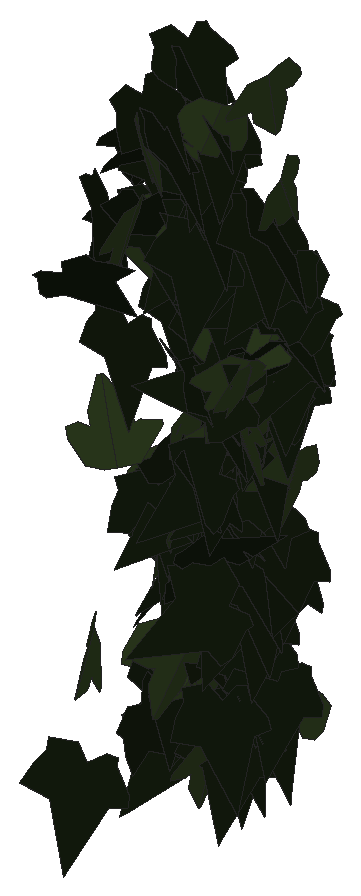
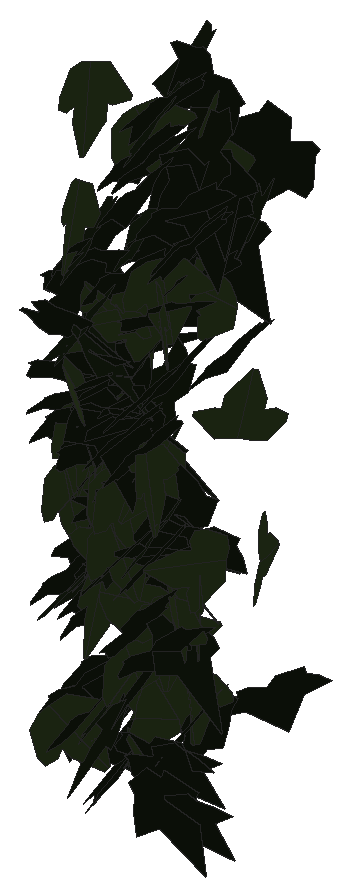
# SketchUp Ruby script. Lengths in inches.
U = 1.inch
M = Sketchup.active_model
def pt(a) = Geom::Point3d.new(a.map { |v| v * U })
def face(e, loops, mat)
  f = e.add_face(loops[0].map { |a| pt(a) })
  loops[1..].each { |l| e.add_face(l.map { |a| pt(a) }).erase! }
  f.material = f.back_material = mat if mat
  f
end
# faces: each face lists its corners as indices into pts; further lists are holes
def faces(e, pts, list, mat = nil) = list.each { |f| face(e, (f[0].is_a?(Array) ? f : [f]).map { |l| l.map { |i| pts[i] } }, mat) }
# xy, xz, yz: faces in a plane at the given z, y or x. An outline is a flat list of corners, or four numbers for a rectangle; further outlines are holes
def ring(l) = l.size == 4 ? [[l[0], l[1]], [l[2], l[1]], [l[2], l[3]], [l[0], l[3]]] : l.each_slice(2).to_a
def flat(e, list, mat, &to3) = list.each { |f| face(e, (f[0].is_a?(Array) ? f : [f]).map { |l| ring(l).map { |u, v| to3.(u, v) } }, mat) }
def xy(e, z, list, mat = nil) = flat(e, list, mat) { |x, y| [x, y, z] }
def xz(e, y, list, mat = nil) = flat(e, list, mat) { |x, z| [x, y, z] }
def yz(e, x, list, mat = nil) = flat(e, list, mat) { |y, z| [x, y, z] }
def lines(e, pts, list) = list.each { |a, b| e.add_line(pt(pts[a]), pt(pts[b])) }
# prism: a flat outline (further loops are holes) pulled along v
def prism(e, loops, v, mat = nil)
  f = face(e, loops, mat); d = Geom::Vector3d.new(v.map { |x| x * U })
  f.pushpull(f.normal.samedirection?(d) ? d.length : -d.length)
end
def box(e, o, s, mat = nil) = prism(e, [[o, [o[0] + s[0], o[1], o[2]], [o[0] + s[0], o[1] + s[1], o[2]], [o[0], o[1] + s[1], o[2]]]], [0, 0, s[2]], mat)
def at(x, y, z, deg = 0) = Geom::Transformation.translation(pt([x, y, z])) * Geom::Transformation.rotation(ORIGIN, Z_AXIS, deg.degrees)
def axes(o, x, y, z) = Geom::Transformation.new([*x, 0, *y, 0, *z, 0, *pt(o).to_a, 1])
def part(name) = M.definitions.add(name)
# library, detail: a bought-in or finely detailed component or shape, given as its bounding box
def library(name, o, s) = part(name).tap { |d| box(d.entities, o, s) }
def detail(e, o, s) = box(e.add_group.entities, o, s)
def put(e, d, t, mat = nil) = e.add_instance(d, t).tap { |i| i.material = mat if mat }
def group(e, t, mat = nil) = e.add_group.tap { |g| g.transformation = t; g.material = mat if mat }.entities
root = M.entities
M.materials.add("efeu1").color = [18, 25, 13]
M.materials.add("efeu2").color = [43, 57, 29]
c1 = part("ivyleaf_9")
p = [[1.54,2.16,1.25],[1.36,2.04,1.19],[-0.21,0.99,0.68],[-0.71,1.11,0.82],[-0.85,0.86,0.67],[-0.8,0.17,0.21],
  [-0.9,-0.01,0.1],[-0.67,-0.16,-0.02],[-0.08,-0.08,-0.05],[-0.03,-0.6,-0.4],[0.65,-0.88,-0.66],[0.83,-0.6,-0.49],
  [1.29,-0.42,-0.43],[1.8125,-0.07,-0.26],[1.21,0.44,0.15]]
faces(c1.entities,p,[[0,1,2,3,4,5,6,7,8,9,10,11,12,13,14]],"efeu1")
c2 = part("ivyleaf_10")
p = [[0,0.5,-0.03],[-0.0625,2.02,-0.43],[-0.19,2.01,-0.46],[-0.54,1.05,-0.29],[-0.52,0.625,-0.18],[-0.83,0.76,-0.28],
  [-1.16,0.64,-0.33],[-1.15,0.33,-0.24],[-0.77,-0.39,0.02],[-0.3,-0.51,0.16],[0.04,-0.48,0.23],[-0.02,2.01,-0.4375],
  [-0.06,2.01,-0.43],[0.04,-0.49,0.23],[0.67,-0.49,0.14],[1.38,0.36,-0.2],[1.375,0.51,-0.24],[0.81,0.65,-0.19],
  [0.62,0.59,-0.15],[0.6,1.09,-0.28],[0.5,1.23,-0.31]]
faces(c2.entities,p,[[0,1,2,3,4,5,6,7,8,9,10],[11,12,0,13,14,15,16,17,18,19,20]],"efeu2")
put(root,c1,axes([13.8,220.49,231.59],[0.40217,0.29091,0.06026],[0.04847,0.03581,-0.49636],[-0.2931,0.40508,0.0006]))
put(root,c2,axes([13.58,221.33,225.61],[-0.05871,0.16785,-0.46731],[0.09367,-0.45837,-0.17641],[-0.48763,-0.10826,0.02238]))
put(root,c1,axes([13.43,221.35,223.65],[-0.19492,-0.45767,-0.05048],[0.01902,0.04677,-0.49744],[0.46005,-0.19584,-0.00082]))
put(root,c1,axes([14.31,221.9375,233.21],[0.2577,-0.40771,0.13176],[0.06772,-0.11306,-0.48232],[0.42309,0.26643,-0.00305]))
put(root,c2,axes([13.76,221.86,231.8],[0.12939,-0.48149,0.03781],[0.01026,-0.0364,-0.49857],[0.48286,0.1298,0.00046]))
put(root,c1,axes([14.9375,222.37,226.15],[-0.39937,-0.19145,0.23205],[-0.21041,-0.09789,-0.44289],[0.21501,-0.4514,-0.00238]))
put(root,c1,axes([12.92,222.48,231.29],[0.01902,-0.28272,0.41195],[0.05223,-0.40887,-0.28302],[0.4969,0.0538,0.01398]))
put(root,c2,axes([13.3,222.09,228.09],[0.35478,0.34849,0.05186],[-0.03906,-0.03425,0.49729],[0.35015,-0.35691,0.00292]))
put(root,c1,axes([13.72,222.21,233.43],[-0.10131,-0.11608,-0.47567],[0.43069,0.20993,-0.14296],[0.23291,-0.4387,0.05745]))
put(root,c2,axes([13.75,222.17,232.93],[-0.27113,0.40326,0.11775],[-0.0681,0.0961,-0.48593],[-0.41455,-0.27954,0.00281]))
put(root,c1,axes([13.07,222.68,229.56],[0.02778,-0.49386,0.07302],[0.02494,-0.07167,-0.49421],[0.4986,0.0311,0.02065]))
put(root,c1,axes([14.53,222.69,227.84],[-0.49906,0.01137,0.02846],[-0.02831,0.00672,-0.49915],[-0.01173,-0.49983,-0.00606]))
put(root,c1,axes([14.83,222.87,229.07],[-0.32268,0.03658,0.38018],[-0.34474,-0.24216,-0.26929],[0.16443,-0.43592,0.1815]))
put(root,c1,axes([14.16,222.89,231.09],[-0.08668,-0.49241,0.00475],[-0.00072,-0.0047,-0.49998],[0.49243,-0.08668,0.0001]))
put(root,c2,axes([14.82,222.86,229.375],[-0.12898,-0.42351,0.23239],[-0.01836,-0.23606,-0.44039],[0.48273,-0.12213,0.04534]))
put(root,c2,axes([13.875,222.85,224.9],[-0.13773,-0.43388,0.20682],[-0.0089,-0.2128,-0.45237],[0.48057,-0.12829,0.05089]))
put(root,c1,axes([13.18,222.78,231.4],[-0.01059,0.33099,-0.37461],[-0.03271,-0.37435,-0.32984],[-0.49882,0.01752,0.02958]))
put(root,c1,axes([14.3125,222.82,229.18],[0.24712,-0.43369,-0.02911],[-0.0123,0.0265,-0.49915],[0.43449,0.24742,0.00243]))
put(root,c1,axes([14.36,222.34,226.53],[0.02979,0.31156,-0.38992],[-0.03442,0.39097,0.30977],[0.49792,0.00839,0.04475]))
put(root,c1,axes([14.48,222.91,224.27],[-0.01662,-0.48072,-0.13651],[0.01341,0.1361,-0.48093],[0.49954,-0.01964,0.00837]))
put(root,c1,axes([14.125,223.16,227.42],[0.03693,-0.39453,0.30493],[0.08476,-0.29635,-0.39369],[0.49138,0.08077,0.04499]))
put(root,c2,axes([14.82,222.96,229.27],[0.10134,-0.48408,0.07345],[0.04823,-0.06477,-0.49344],[0.48724,0.10709,0.03356]))
put(root,c1,axes([13.14,222.84,232.71],[0.45503,-0.16343,0.12743],[0.12074,-0.04079,-0.48348],[0.16842,0.47077,0.00234]))
put(root,c2,axes([14.2,223.11,232.9],[-0.27405,-0.36356,0.2067],[-0.03242,-0.22791,-0.44385],[0.41695,-0.25668,0.10134]))
put(root,c1,axes([13.32,222.7,223.94],[0.12955,-0.17125,-0.45154],[-0.27108,0.36112,-0.21473],[0.39967,0.30044,0.00072]))
put(root,c2,axes([14.22,223,223.52],[-0.00411,-0.49998,0.00247],[0.00009,-0.00247,-0.49999],[0.49998,-0.00411,0.00011]))
put(root,c1,axes([14.42,223.29,225.77],[-0.15318,-0.46276,0.11131],[-0.00387,-0.11572,-0.48641],[0.47594,-0.14987,0.03187]))
put(root,c1,axes([13.64,223.17,228.84],[0.2707,-0.28854,0.30573],[0.20662,-0.22535,-0.39563],[0.3661,0.34053,-0.00277]))
put(root,c1,axes([13.97,223.33,232.49],[-0.07643,-0.4726,0.14423],[0.01277,-0.14779,-0.47749],[0.49396,-0.0693,0.03466]))
put(root,c1,axes([14.39,223.21,230.55],[-0.07448,-0.48829,-0.07762],[0.01205,0.07668,-0.49394],[0.49427,-0.07545,0.00035]))
put(root,c1,axes([13.98,223.13,226.47],[-0.46616,0.15472,-0.09356],[0.07969,-0.05644,-0.49037],[-0.16231,-0.4721,0.02796]))
put(root,c1,axes([14.8,223.07,229.54],[-0.05792,0.39795,-0.29712],[-0.01346,-0.30028,-0.39956],[-0.49645,-0.03828,0.0455]))
put(root,c1,axes([13.9375,223.37,231.42],[0.12592,-0.42098,0.23857],[0.09317,-0.22081,-0.43882],[0.47483,0.15497,0.02283]))
put(root,c1,axes([13.22,222.99,232.48],[0.14415,0.41585,-0.23726],[-0.11216,-0.21156,-0.43894],[-0.46545,0.17977,0.03229]))
put(root,c1,axes([13.2,223.1875,226.9375],[-0.22781,-0.27437,-0.35046],[0.25165,0.24533,-0.35565],[0.36712,-0.33843,0.02632]))
put(root,c2,axes([12.81,223.1875,230.6875],[0.03293,-0.00362,-0.4989],[0.48507,-0.11672,0.03286],[-0.11671,-0.48617,-0.00418]))
put(root,c1,axes([14.33,223.4,223.53],[-0.1431,-0.47844,-0.0248],[0.00712,0.02375,-0.49938],[0.47903,-0.14328,0.00002]))
put(root,c2,axes([14.54,223.125,228.58],[-0.42208,0.24059,-0.11818],[0.11016,-0.04527,-0.48561],[-0.24437,-0.43597,-0.01479]))
put(root,c1,axes([13.16,223.02,232.26],[0.02208,0.48811,-0.10612],[-0.0255,-0.10498,-0.48819],[-0.49886,0.02697,0.02025]))
put(root,c1,axes([13.13,223.47,224.07],[0.0721,-0.47323,0.14443],[0.01853,-0.14327,-0.47868],[0.49443,0.07438,-0.00313]))
put(root,c1,axes([13.625,223.48,226.87],[-0.43349,-0.22149,0.11413],[-0.08849,-0.07725,-0.48601],[0.23293,-0.44156,0.02777]))
put(root,c1,axes([13.6,223.47,226.4],[-0.23787,-0.43953,-0.01522],[0.00627,0.01391,-0.49977],[0.43975,-0.23795,-0.0011]))
put(root,c2,axes([13.33,223.48,226.14],[0.1681,-0.30768,0.35648],[0.23999,-0.26969,-0.34594],[0.40515,0.28741,0.05702]))
put(root,c2,axes([14.22,223.02,229.86],[-0.00451,-0.13108,-0.48249],[0.43338,0.23958,-0.06914],[0.24931,-0.41883,0.11145]))
put(root,c1,axes([13.01,223.39,231.07],[0.03277,-0.48026,-0.1352],[0.00898,0.13604,-0.48105],[0.49884,0.0291,0.01754]))
put(root,c1,axes([13.97,223.51,232.7],[0.00664,-0.49941,0.02346],[0.00257,-0.02343,-0.49944],[0.49995,0.00676,0.00225]))
put(root,c1,axes([13.66,223.47,233.3],[0.23133,-0.44022,0.0519],[0.01667,-0.04986,-0.49723],[0.44295,0.23178,-0.00839]))
put(root,c2,axes([14.54,223.15,229.6],[0.44429,0.0906,-0.21072],[0.18189,0.14069,0.44399],[0.13974,-0.47117,0.09205]))
put(root,c2,axes([13.21,223.35,224.625],[0.4042,0.29343,-0.0228],[-0.01842,-0.01343,-0.49948],[-0.29374,0.40462,-0.00005]))
put(root,c1,axes([14.61,223.625,225.58],[-0.00863,-0.48833,0.10704],[-0.009,-0.10689,-0.48836],[0.49984,-0.01036,-0.00695]))
put(root,c1,axes([14.47,223.47,226.4],[0.20512,-0.45452,-0.03653],[-0.01286,0.03428,-0.49866],[0.45581,0.20551,0.00237]))
put(root,c1,axes([13.52,223.42,233.67],[0.12425,-0.46195,-0.14548],[0.0302,0.15729,-0.47365],[0.48337,0.10892,0.06699]))
put(root,c2,axes([13.12,223.27,226.23],[0.26637,-0.35799,-0.22559],[-0.05657,0.23404,-0.43821],[0.41934,0.25897,0.08418]))
put(root,c1,axes([13.16,223.69,229.68],[0.07704,-0.48639,0.08656],[0.01603,-0.0851,-0.49244],[0.49377,0.07865,0.00248]))
put(root,c2,axes([13.97,223.62,224.86],[-0.18934,-0.43701,0.15222],[-0.01224,-0.15968,-0.47366],[0.4626,-0.18309,0.04978]))
put(root,c1,axes([14.99,223.86,230.32],[-0.25434,-0.23956,0.35766],[-0.26721,-0.23784,-0.34932],[0.33751,-0.36884,-0.00704]))
put(root,c1,axes([12.88,223.68,231.85],[0.05867,-0.49537,-0.0341],[0.00406,0.03481,-0.49877],[0.49653,0.05825,0.00811]))
put(root,c1,axes([13.09,223.7,232.24],[-0.08759,-0.48806,-0.06424],[0.00979,0.06351,-0.49585],[0.49217,-0.08812,-0.00157]))
put(root,c1,axes([14.82,223.83,230.78],[-0.30877,-0.37835,0.1073],[-0.04319,-0.10297,-0.48737],[0.39089,-0.31024,0.03091]))
put(root,c1,axes([14.4,223.78,227.33],[-0.43744,-0.19281,0.14653],[-0.1209,-0.08828,-0.47706],[0.20983,-0.45281,0.03061]))
put(root,c1,axes([13.8,223.7,232.29],[0.06384,-0.49524,-0.02571],[-0.00083,0.02582,-0.49933],[0.49591,0.0638,0.00248]))
put(root,c1,axes([14.57,223.73,231.27],[0.01078,-0.49938,-0.02236],[-0.01016,0.02214,-0.49941],[0.49978,0.01122,-0.00967]))
put(root,c2,axes([14.82,223.46,233.5],[-0.12814,-0.46412,-0.13481],[0.02634,0.13256,-0.48139],[0.48258,-0.13047,-0.00953]))
put(root,c1,axes([14.44,223.71,225.98],[0.03777,-0.49587,-0.05183],[0.00194,0.05212,-0.49727],[0.49857,0.03736,0.00586]))
put(root,c1,axes([14.3125,223.73,224.88],[-0.04806,-0.48879,-0.09366],[0.00931,0.0932,-0.49115],[0.4976,-0.04896,0.00015]))
put(root,c2,axes([13.52,223.875,224.29],[0.01584,0.20118,-0.45747],[-0.18745,-0.42189,-0.19203],[-0.46326,0.17759,0.06206]))
put(root,c1,axes([13.47,223.79,227.07],[0.18622,-0.4485,0.11902],[0.04437,-0.11045,-0.48563],[0.4619,0.19143,-0.00134]))
put(root,c1,axes([13.33,223.36,227.04],[0.07028,-0.00591,0.495],[0.47915,0.12645,-0.06652],[-0.1244,0.48371,0.02343]))
put(root,c1,axes([13.66,223.5,224.92],[0.26332,-0.33557,-0.26087],[-0.13906,0.22198,-0.4259],[0.40165,0.29685,0.02357]))
put(root,c2,axes([14.14,223.68,225.9],[0.05906,0.01763,-0.49619],[-0.4942,-0.04594,-0.06045],[-0.04772,0.49757,0.012]))
put(root,c1,axes([13.22,223.53,225.54],[-0.21933,0.43648,-0.10667],[0.01729,-0.11042,-0.48735],[-0.44899,-0.21747,0.03335]))
put(root,c1,axes([13.39,223.95,230.59],[-0.33004,-0.35694,0.1169],[0.00234,-0.15757,-0.47452],[0.37559,-0.31268,0.10568]))
put(root,c1,axes([14.0625,223.75,227.49],[-0.03503,-0.48074,-0.13289],[0.0501,0.12916,-0.48043],[0.49625,-0.04697,0.03912]))
put(root,c1,axes([14.7,223.89,224.36],[-0.10382,-0.4889,0.0141],[-0.00248,-0.01389,-0.4998],[0.4891,-0.10385,0.00046]))
put(root,c1,axes([13.99,223.93,223.28],[0.08024,-0.46634,0.16152],[0.01253,-0.16166,-0.47298],[0.49336,0.07995,-0.01425]))
put(root,c1,axes([13.12,223.875,223.02],[-0.44422,-0.2295,0.00212],[-0.00164,-0.00143,-0.5],[0.2295,-0.44422,0.00052]))
put(root,c2,axes([13.36,223.58,225.77],[-0.49094,-0.01072,0.09416],[-0.09429,0.00527,-0.491],[0.00953,-0.49986,-0.0072]))
put(root,c1,axes([13.58,223.96,229.22],[-0.01071,-0.4769,0.14984],[0.0416,-0.1502,-0.47509],[0.49815,0.00229,0.04289]))
put(root,c1,axes([14.53,223.79,231.34],[0.27326,-0.41605,0.04726],[0.01506,-0.04663,-0.49759],[0.41845,0.27337,-0.01295]))
put(root,c1,axes([14.4,223.9,227.8],[0.11736,-0.47512,0.10238],[0.03183,-0.09759,-0.48935],[0.48499,0.12138,0.00734]))
put(root,c1,axes([14.61,223.72,229.77],[-0.39206,0.29048,-0.10915],[0.05707,-0.10538,-0.48543],[-0.30501,-0.39309,0.04948]))
put(root,c2,axes([14.02,223.83,227.73],[-0.28066,-0.37112,0.18302],[-0.04172,-0.19465,-0.45866],[0.41169,-0.27273,0.07829]))
put(root,c1,axes([14.625,223.98,228.61],[-0.42637,-0.24126,0.10001],[-0.0508,-0.11119,-0.48483],[0.25618,-0.42359,0.07031]))
put(root,c1,axes([13.93,224.01,226.64],[-0.33682,-0.3631,0.06865],[-0.00063,-0.09232,-0.4914],[0.36953,-0.33111,0.06173]))
put(root,c2,axes([12.82,223.35,226.7],[0.01852,0.04871,-0.49728],[0.294,0.40129,0.05026],[0.404,-0.29426,-0.01378]))
put(root,c1,axes([14.3125,223.96,228.6],[-0.11677,-0.48596,0.0144],[-0.01172,-0.01199,-0.49972],[0.48603,-0.11704,-0.00859]))
put(root,c1,axes([14.32,223.77,226.75],[-0.11951,-0.4109,-0.25862],[0.07997,0.24604,-0.42787],[0.47888,-0.14363,0.00691]))
put(root,c1,axes([12.78,223.86,231.86],[0.11637,-0.48047,-0.07486],[-0.00519,0.07574,-0.4942],[0.48624,0.1158,0.01264]))
put(root,c2,axes([13.56,223.49,228.1],[-0.10261,-0.32946,-0.36184],[0.14529,0.33253,-0.34397],[0.46729,-0.17573,0.0275]))
put(root,c1,axes([14.07,223.625,226.6875],[0.43188,-0.22495,-0.11347],[-0.05725,0.13167,-0.47894],[0.24535,0.42669,0.08798]))
put(root,c2,axes([14.25,223.6875,228.6],[-0.45999,-0.18522,-0.0641],[0.0585,0.02633,-0.49587],[0.18706,-0.46368,-0.00255]))
put(root,c1,axes([14.5,223.88,224.01],[0.08757,-0.48469,-0.08607],[-0.01957,0.08392,-0.49252],[0.49188,0.08963,-0.00427]))
put(root,c1,axes([13.22,224.02,223.81],[-0.43498,-0.24522,0.02564],[-0.02247,-0.01236,-0.49934],[0.24553,-0.43556,-0.00027]))
put(root,c1,axes([14.8125,224.08,229.42],[-0.33994,-0.36666,0.00079],[0.056,-0.05298,-0.49402],[0.36236,-0.33579,0.07709]))
put(root,c1,axes([14.21,223.65,224.12],[0.40294,-0.14969,-0.25541],[-0.22789,0.1185,-0.42898],[0.18896,0.46211,0.02728]))
put(root,c1,axes([14.65,224.16,225.95],[-0.04895,-0.41588,0.27322],[0.06452,-0.27753,-0.41087],[0.4934,-0.00497,0.08083]))
put(root,c1,axes([13.6,224.21,225.73],[-0.18554,-0.34655,0.30899],[-0.0977,-0.29616,-0.39082],[0.45391,-0.2054,0.04219]))
put(root,c1,axes([14.54,223.85,230.07],[0.30917,-0.38808,-0.06173],[-0.00582,0.07401,-0.49446],[0.39291,0.30646,0.04125]))
put(root,c2,axes([13.22,223.91,231.22],[-0.36911,-0.32634,0.0852],[0.00701,-0.1337,-0.48174],[0.3372,-0.35444,0.10328]))
put(root,c1,axes([13.82,223.9375,228.61],[0.12426,-0.47795,-0.07827],[0.01517,0.0846,-0.49256],[0.48408,0.12003,0.03553]))
put(root,c2,axes([13.85,223.95,227.6875],[-0.20201,-0.44429,0.10863],[0.02114,-0.1277,-0.48296],[0.45689,-0.19053,0.07037]))
put(root,c1,axes([13.86,223.97,223.52],[0.16845,-0.46881,-0.04288],[-0.01071,0.04171,-0.49814],[0.47065,0.16874,0.00401]))
put(root,c2,axes([14.39,223.71,225.98],[-0.02638,-0.43565,-0.24394],[0.05084,0.24067,-0.43531],[0.49671,-0.04777,0.0316]))
put(root,c1,axes([14.67,224.13,226.28],[-0.03332,-0.49542,0.05869],[0.00518,-0.05916,-0.49646],[0.49886,-0.03248,0.00907]))
put(root,c1,axes([13.28,224.06,224.01],[-0.39754,-0.25166,-0.16922],[0.16474,0.05503,-0.46886],[0.25461,-0.42853,0.03917]))
put(root,c1,axes([14.13,223.72,228.84],[0.08879,0.46068,-0.17289],[-0.08889,-0.15778,-0.46605],[-0.48396,0.1135,0.05388]))
put(root,c2,axes([13.49,223.85,228.24],[0.07923,-0.48306,-0.10188],[-0.02362,0.09936,-0.48946],[0.49312,0.08237,-0.00707]))
put(root,c2,axes([13.34,223.84,230.88],[0.30776,-0.3712,-0.13226],[-0.04593,0.13289,-0.47982],[0.39137,0.30749,0.0477]))
put(root,c2,axes([14.82,223.96,227.55],[-0.08902,-0.48914,0.05311],[0.00344,-0.05459,-0.497],[0.492,-0.08813,0.01308]))
put(root,c1,axes([13.43,224.04,228.56],[0.09739,-0.48852,-0.04319],[-0.00912,0.04222,-0.49813],[0.49034,0.09781,-0.00069]))
put(root,c1,axes([13.18,223.92,223.43],[-0.148,0.3929,-0.27152],[0.09731,-0.25349,-0.41985],[-0.46757,-0.17712,-0.00144]))
put(root,c2,axes([14.06,223.93,226.82],[-0.09124,-0.49029,0.03591],[0.02918,0.03106,0.49818],[-0.49074,0.093,0.02294]))
put(root,c2,axes([14.75,223.88,228.43],[-0.02645,-0.49427,-0.07072],[0.01343,0.07009,-0.49488],[0.49912,-0.02808,0.00957]))
put(root,c1,axes([14.57,224.15,229.09],[-0.10066,-0.48892,-0.02868],[0.11257,0.0054,-0.48713],[0.47665,-0.10453,0.10899]))
put(root,c1,axes([13.125,224.22,225.61],[-0.18548,-0.45683,0.08308],[-0.00561,-0.08725,-0.4923],[0.46429,-0.18355,0.02724]))
put(root,c1,axes([14.24,224.24,228.46],[-0.2255,-0.43273,0.10904],[-0.05327,-0.09519,-0.48796],[0.44307,-0.23169,-0.00317]))
put(root,c2,axes([14.79,224.14,223.91],[-0.27535,-0.25586,0.32973],[-0.14564,-0.31129,-0.36317],[0.39111,-0.29604,0.0969]))
put(root,c1,axes([15.08,224.11,230.08],[-0.48758,-0.04456,0.1014],[-0.0974,-0.04546,-0.48831],[0.05274,-0.49593,0.03565]))
put(root,c1,axes([13.98,224.01,224.49],[0.25593,-0.42849,-0.02999],[-0.01083,0.02846,-0.49907],[0.4294,0.2561,0.00529]))
put(root,c2,axes([14.36,224.12,228.46],[0.29847,-0.30076,0.26545],[0.19828,-0.17701,-0.4235],[0.34872,0.35807,0.0136]))
put(root,c2,axes([14.78,223.76,231.8125],[0.06203,-0.41768,-0.26777],[0.02345,0.27202,-0.41888],[0.49558,0.03941,0.05333]))
put(root,c2,axes([14.58,224.15,229.3125],[0.26747,-0.33995,0.2508],[0.14432,-0.20545,-0.43239],[0.39703,0.30369,-0.01178]))
put(root,c1,axes([14.58,224.14,228.82],[-0.03059,-0.49632,-0.05231],[-0.0041,0.05265,-0.4972],[0.49905,-0.02999,-0.00729]))
put(root,c2,axes([13.89,224.08,227.05],[-0.1737,-0.44712,0.14111],[-0.0293,-0.13983,-0.47915],[0.46794,-0.17473,0.02237]))
put(root,c1,axes([13.21,224.11,226.96],[0.15318,-0.47596,-0.00104],[0.01498,0.00592,-0.49974],[0.47572,0.15307,0.01608]))
put(root,c1,axes([13.82,224.35,226.66],[-0.10601,-0.39896,0.28212],[0.02121,-0.29217,-0.4052],[0.48817,-0.07394,0.07887]))
